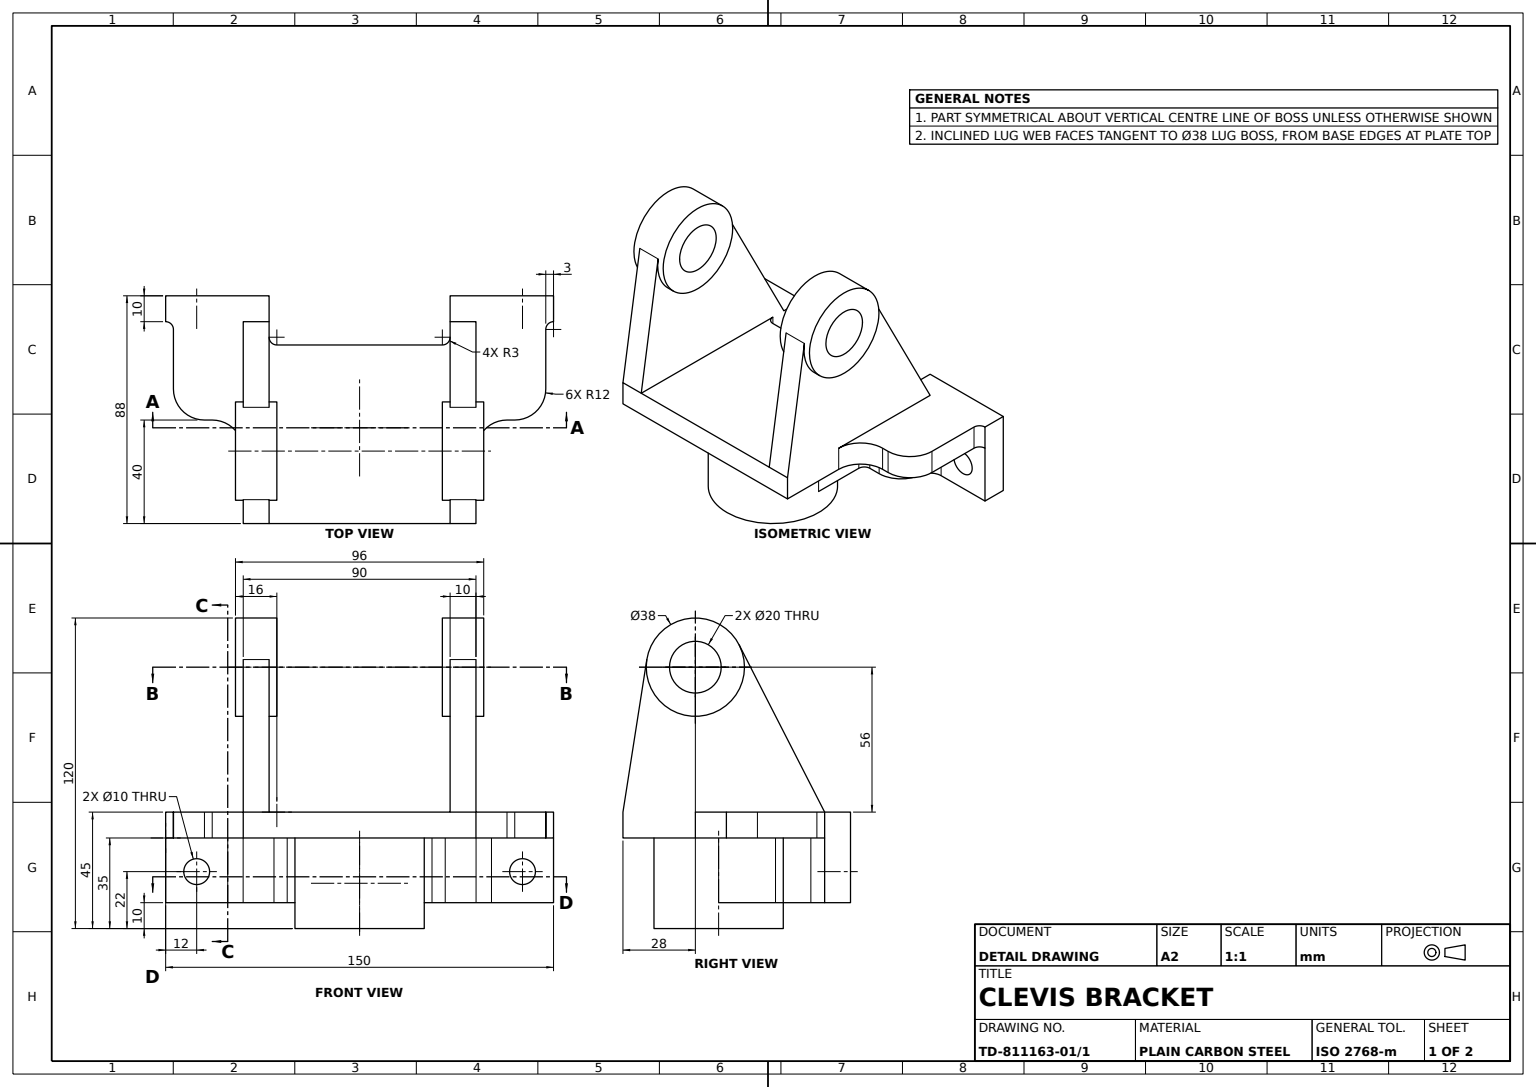
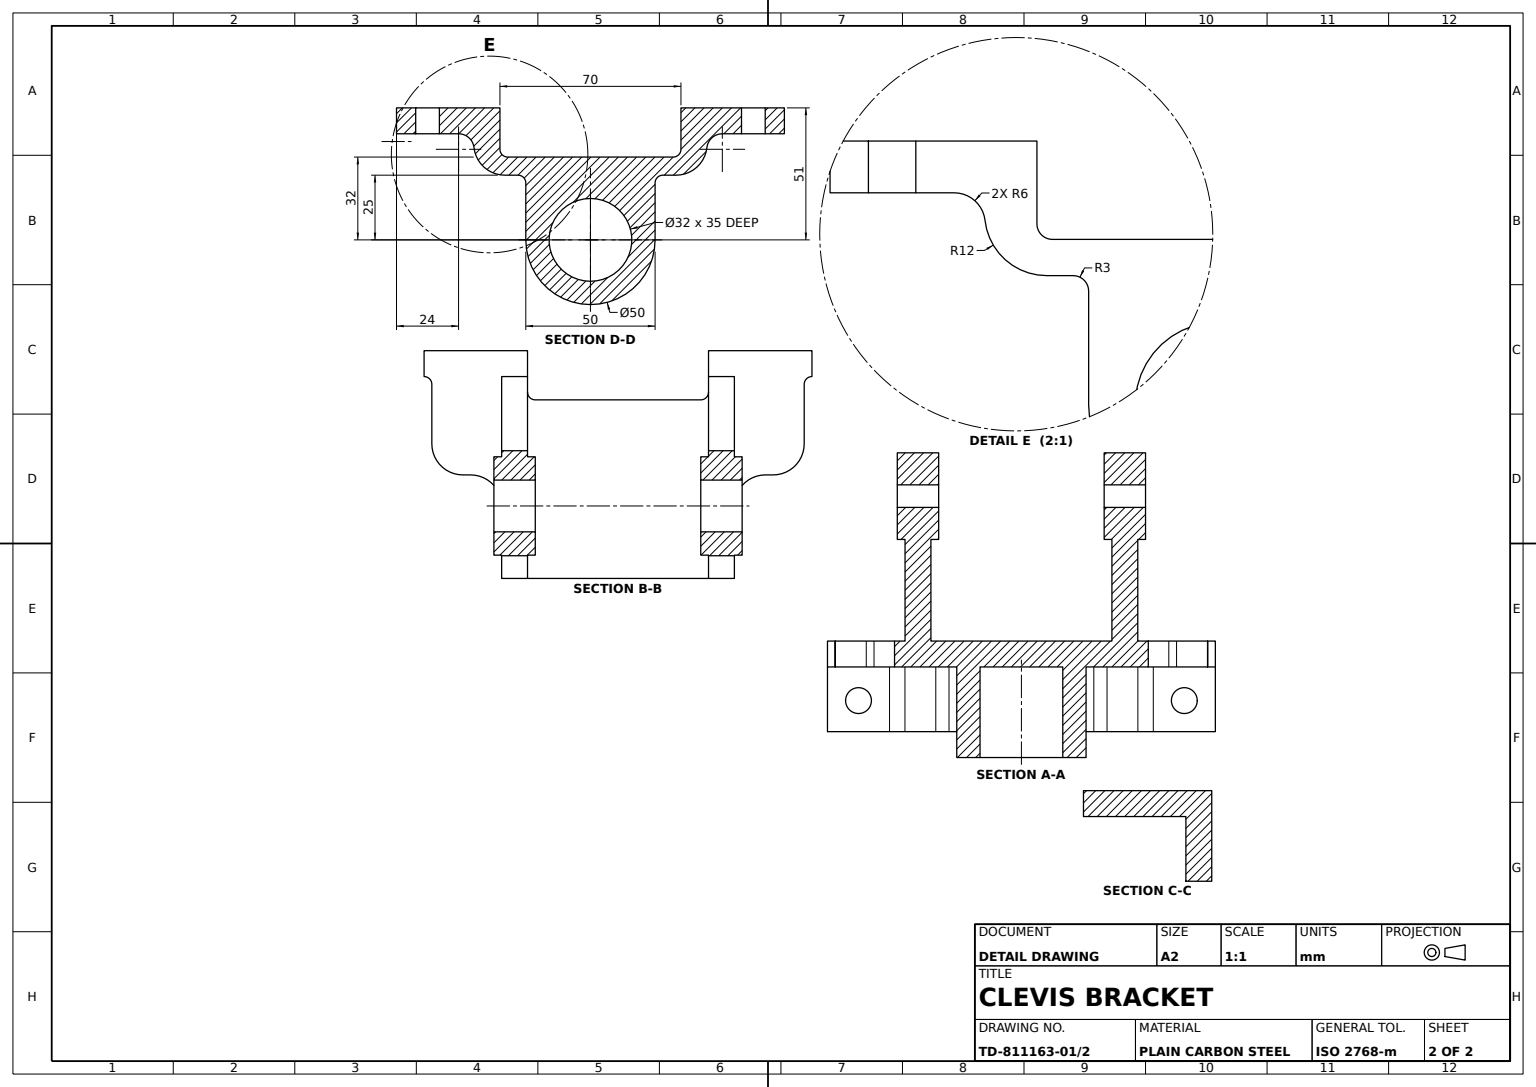
solid
v1 (48,101,19)
v2 (32,101,19)
e1 v1 v2 LINE
v3 (48,101,-1)
e2 v3 v1 CIRCLE(AX(P(48,101,9),D(-1,0,0),D(0,0,1)),10)
v4 (32,101,-1)
e3 v3 v4 LINE
e4 v4 v2 CIRCLE(AX(P(32,101,9),D(-1,0,0),D(0,0,1)),10)
face CYL(AX(P(75,101,9),D(-1,0,0),D(0,0,1)),10) rev [-e1 -e2 e3 e4]
v5 (-45.037152,10,-35.666667)
v6 (-45.037152,35,-35.666667)
e5 v5 v6 LINE
v7 (-51,35,-41)
e6 v7 v6 CIRCLE(AX(P(-51,35,-35),D(0,-1,0),D(0,0,1)),6)
v8 (-51,10,-41)
e7 v8 v7 LINE
e8 v8 v5 CIRCLE(AX(P(-51,10,-35),D(0,-1,0),D(0,0,1)),6)
face CYL(AX(P(-51,10,-35),D(0,1,0),D(0,0,1)),6) rev [e5 -e6 -e7 e8]
v9 (-68,22,-41)
v10 (-58,22,-41)
e9 v9 v10 CIRCLE(AX(P(-63,22,-41),D(0,0,1),D(1,0,0)),5)
e10 v10 v9 CIRCLE(AX(P(-63,22,-41),D(0,0,1),D(1,0,0)),5)
v11 (-75,10,-41)
e11 v11 v8 LINE
v12 (-75,35,-41)
e12 v12 v7 LINE
e13 v11 v12 LINE
face PLANE(AX(P(-51,10,-41),D(0,0,1),D(1,0,0))) [-e9 -e10] [e11 e7 -e12 -e13]
v13 (-48,101,-1)
v14 (-48,101,19)
e14 v13 v14 CIRCLE(AX(P(-48,101,9),D(-1,0,0),D(0,0,1)),10)
e15 v14 v13 CIRCLE(AX(P(-48,101,9),D(-1,0,0),D(0,0,1)),10)
v15 (-48,101,28)
v16 (-48,101,-10)
e16 v15 v16 CIRCLE(AX(P(-48,101,9),D(1,0,0),D(0,0,-1)),19)
e17 v16 v15 CIRCLE(AX(P(-48,101,9),D(1,0,0),D(0,0,-1)),19)
face PLANE(AX(P(-48,0,0),D(1,0,0),D(0,0,-1))) rev [-e14 -e15] [-e16 -e17]
v17 (32,45,-32)
v18 (-32,45,-32)
e18 v17 v18 LINE
v19 (-35,45,-35)
e19 v18 v19 CIRCLE(AX(P(-32,45,-35),D(0,-1,0),D(0,0,1)),3)
v20 (-35,45,37)
e20 v20 v19 LINE
v21 (35,45,37)
e21 v20 v21 LINE
v22 (35,45,-35)
e22 v21 v22 LINE
e23 v22 v17 CIRCLE(AX(P(32,45,-35),D(0,-1,0),D(0,0,1)),3)
face PLANE(AX(P(-57,45,9),D(0,-1,0),D(0,0,-1))) rev [e18 e19 -e20 e21 e22 e23]
v23 (-75,45,-41)
v24 (-72,45,-38)
e24 v23 v24 CIRCLE(AX(P(-75,45,-38),D(0,-1,0),D(0,0,-1)),3)
e25 v12 v23 LINE
v25 (-72,35,-38)
e26 v25 v12 CIRCLE(AX(P(-75,35,-38),D(0,1,0),D(0,0,-1)),3)
e27 v24 v25 LINE
face CYL(AX(P(-75,45,-38),D(0,-1,0),D(0,0,-1)),3) rev [-e24 -e25 -e26 -e27]
v26 (-25,10,0)
v27 (0,10,-25)
e28 v26 v27 CIRCLE(AX(P(0,10,0),D(0,-1,0),D(0,0,1)),25)
v28 (0,0,-25)
e29 v27 v28 LINE
v29 (0,0,25)
e30 v28 v29 CIRCLE(AX(P(0,0,0),D(0,1,0),D(0,0,1)),25)
v30 (0,35,25)
e31 v30 v29 LINE
v31 (-25,35,0)
e32 v31 v30 CIRCLE(AX(P(0,35,0),D(0,1,0),D(0,0,1)),25)
e33 v26 v31 LINE
face CYL(AX(P(0,35,0),D(0,-1,0),D(0,0,-1)),25) [e28 e29 e30 -e31 -e32 -e33]
v32 (28,10,-25)
v33 (33.111456,10,-25)
e34 v32 v33 LINE
v34 (33.111456,35,-25)
e35 v33 v34 LINE
v35 (28,35,-25)
e36 v35 v34 LINE
e37 v32 v35 LINE
face PLANE(AX(P(45,10,-25),D(0,0,1),D(1,0,0))) [e34 e35 -e36 -e37]
v36 (58,22,-51)
v37 (68,22,-51)
e38 v36 v37 CIRCLE(AX(P(63,22,-51),D(0,0,1),D(1,0,0)),5)
e39 v37 v36 CIRCLE(AX(P(63,22,-51),D(0,0,1),D(1,0,0)),5)
v38 (75,45,-51)
v39 (35,45,-51)
e40 v38 v39 LINE
v40 (75,10,-51)
e41 v40 v38 LINE
v41 (35,10,-51)
e42 v40 v41 LINE
e43 v41 v39 LINE
face PLANE(AX(P(35,10,-51),D(0,0,-1),D(-1,0,0))) [e38 e39] [-e40 -e41 e42 e43]
e44 v29 v28 CIRCLE(AX(P(0,0,0),D(0,1,0),D(0,0,1)),25)
v42 (0,0,-16)
v43 (0,0,16)
e45 v42 v43 CIRCLE(AX(P(0,0,0),D(0,-1,0),D(0,0,-1)),16)
e46 v43 v42 CIRCLE(AX(P(0,0,0),D(0,-1,0),D(0,0,-1)),16)
face PLANE(AX(P(0,0,0),D(0,1,0),D(0,0,1))) rev [-e30 -e44] [-e45 -e46]
v44 (-25,10,-22)
v45 (-25,35,-22)
e47 v44 v45 LINE
v46 (-28,35,-25)
e48 v46 v45 CIRCLE(AX(P(-28,35,-22),D(0,-1,0),D(0,0,1)),3)
v47 (-28,10,-25)
e49 v47 v46 LINE
e50 v47 v44 CIRCLE(AX(P(-28,10,-22),D(0,-1,0),D(0,0,1)),3)
face CYL(AX(P(-28,10,-22),D(0,1,0),D(0,0,1)),3) rev [e47 -e48 -e49 e50]
v48 (48,101,28)
v49 (48,101,-10)
e51 v48 v49 CIRCLE(AX(P(48,101,9),D(1,0,0),D(0,0,-1)),19)
e52 v49 v48 CIRCLE(AX(P(48,101,9),D(1,0,0),D(0,0,-1)),19)
e53 v1 v3 CIRCLE(AX(P(48,101,9),D(-1,0,0),D(0,0,1)),10)
face PLANE(AX(P(48,0,0),D(-1,0,0),D(0,0,-1))) rev [e51 e52] [e53 e2]
v50 (-35,10,-51)
v51 (-35,45,-51)
e54 v50 v51 LINE
v52 (-75,10,-51)
e55 v50 v52 LINE
v53 (-75,45,-51)
e56 v52 v53 LINE
e57 v51 v53 LINE
v54 (-68,22,-51)
v55 (-58,22,-51)
e58 v54 v55 CIRCLE(AX(P(-63,22,-51),D(0,0,1),D(1,0,0)),5)
e59 v55 v54 CIRCLE(AX(P(-63,22,-51),D(0,0,1),D(1,0,0)),5)
face PLANE(AX(P(-75,10,-51),D(0,0,-1),D(-1,0,0))) [-e54 e55 e56 -e57] [e58 e59]
v56 (-33.111456,10,-25)
e60 v56 v47 LINE
v57 (-33.111456,35,-25)
e61 v57 v46 LINE
e62 v57 v56 LINE
face PLANE(AX(P(-28,10,-25),D(0,0,1),D(1,0,0))) [e60 e49 -e61 e62]
v58 (68,22,-41)
v59 (58,22,-41)
e63 v58 v59 CIRCLE(AX(P(63,22,-41),D(0,0,1),D(1,0,0)),5)
e64 v59 v58 CIRCLE(AX(P(63,22,-41),D(0,0,1),D(1,0,0)),5)
v60 (51,10,-41)
v61 (51,35,-41)
e65 v60 v61 LINE
v62 (75,10,-41)
e66 v60 v62 LINE
v63 (75,35,-41)
e67 v62 v63 LINE
e68 v61 v63 LINE
face PLANE(AX(P(75,10,-41),D(0,0,1),D(1,0,0))) [-e63 -e64] [-e65 e66 e67 -e68]
v64 (72,35,-38)
v65 (72,45,-38)
e69 v64 v65 LINE
v66 (72,45,-15)
e70 v66 v65 LINE
v67 (72,35,-15)
e71 v66 v67 LINE
e72 v67 v64 LINE
face PLANE(AX(P(72,45,-41),D(-1,0,0),D(0,0,1))) rev [e69 -e70 e71 e72]
e73 v52 v11 LINE
e74 v53 v23 LINE
face PLANE(AX(P(-75,10,-41),D(-1,0,0),D(0,0,1))) [e73 e13 e25 -e74 -e56]
v68 (35,10,-35)
e75 v41 v68 LINE
e76 v68 v22 LINE
v69 (35,103.939212,27.771282)
e77 v21 v69 LINE
v70 (35,101,28)
e78 v69 v70 CIRCLE(AX(P(35,101,9),D(1,0,0),D(0,0,-1)),19)
v71 (35,101,-10)
e79 v70 v71 CIRCLE(AX(P(35,101,9),D(1,0,0),D(0,0,-1)),19)
v72 (35,109.655382,-7.914028)
e80 v71 v72 CIRCLE(AX(P(35,101,9),D(1,0,0),D(0,0,-1)),19)
v73 (35,45,-41)
e81 v73 v72 LINE
e82 v39 v73 LINE
face PLANE(AX(P(35,10,-35),D(-1,0,0),D(0,0,1))) [-e43 e75 e76 -e22 e77 e78 e79 e80 -e81 -e82]
e83 v45 v31 LINE
e84 v44 v26 LINE
face PLANE(AX(P(-25,10,0),D(-1,0,0),D(0,0,1))) [-e83 -e47 e84 e33]
v74 (-45,101,-10)
e85 v74 v16 LINE
v75 (-45,101,28)
e86 v75 v74 CIRCLE(AX(P(-45,101,9),D(1,0,0),D(0,0,-1)),19)
e87 v75 v15 LINE
face CYL(AX(P(-32,101,9),D(-1,0,0),D(0,0,1)),19) [-e85 -e86 e87 e16]
v76 (-57,45,-3)
v77 (-57,35,-3)
e88 v76 v77 LINE
v78 (-45,35,9)
e89 v77 v78 CIRCLE(AX(P(-57,35,9),D(0,-1,0),D(0,0,-1)),12)
v79 (-45,45,9)
e90 v79 v78 LINE
e91 v76 v79 CIRCLE(AX(P(-57,45,9),D(0,-1,0),D(0,0,-1)),12)
face CYL(AX(P(-57,45,9),D(0,-1,0),D(0,0,-1)),12) rev [e88 e89 -e90 -e91]
e92 v36 v59 LINE
e93 v37 v58 LINE
face CYL(AX(P(63,22,-51),D(0,0,1),D(1,0,0)),5) rev [-e92 -e39 e93 e63]
v80 (-45,45,37)
v81 (-45,103.939212,27.771282)
e94 v80 v81 LINE
e95 v80 v20 LINE
v82 (-35,103.939212,27.771282)
e96 v20 v82 LINE
e97 v82 v81 LINE
face PLANE(AX(P(-35,6.731708,42.99206),D(0,0.154695393,0.987962214),D(0,-0.987962214,0.154695393))) [-e94 e95 e96 e97]
v83 (-35,10,-35)
e98 v83 v19 LINE
e99 v83 v50 LINE
v84 (-35,45,-41)
e100 v84 v51 LINE
v85 (-35,109.655382,-7.914028)
e101 v84 v85 LINE
v86 (-35,101,-10)
e102 v86 v85 CIRCLE(AX(P(-35,101,9),D(1,0,0),D(0,0,-1)),19)
v87 (-35,101,28)
e103 v87 v86 CIRCLE(AX(P(-35,101,9),D(1,0,0),D(0,0,-1)),19)
e104 v82 v87 CIRCLE(AX(P(-35,101,9),D(1,0,0),D(0,0,-1)),19)
face PLANE(AX(P(-35,10,-51),D(1,0,0),D(0,0,-1))) [-e96 e20 -e98 e99 e54 -e100 e101 -e102 -e103 -e104]
v88 (25,10,-22)
v89 (25,35,-22)
e105 v88 v89 LINE
v90 (25,35,0)
e106 v90 v89 LINE
v91 (25,10,0)
e107 v91 v90 LINE
e108 v91 v88 LINE
face PLANE(AX(P(25,10,-22),D(1,0,0),D(0,0,-1))) [e105 -e106 -e107 e108]
v92 (0,35,-16)
e109 v92 v42 LINE
v93 (0,35,16)
e110 v93 v43 LINE
e111 v93 v92 CIRCLE(AX(P(0,35,0),D(0,1,0),D(0,0,-1)),16)
face CYL(AX(P(0,45,0),D(0,-1,0),D(0,0,-1)),16) rev [e109 e45 -e110 e111]
e112 v92 v93 CIRCLE(AX(P(0,35,0),D(0,1,0),D(0,0,-1)),16)
face CYL(AX(P(0,45,0),D(0,-1,0),D(0,0,-1)),16) rev [e112 e110 e46 -e109]
e113 v6 v57 CIRCLE(AX(P(-33.111456,35,-37),D(0,1,0),D(0,0,-1)),12)
e114 v56 v5 CIRCLE(AX(P(-33.111456,10,-37),D(0,-1,0),D(0,0,1)),12)
face CYL(AX(P(-33.111456,10,-37),D(0,1,0),D(0,0,1)),12) [-e62 -e113 -e5 -e114]
v94 (45,45,-41)
e115 v73 v94 LINE
v95 (45,109.655382,-7.914028)
e116 v72 v95 LINE
e117 v94 v95 LINE
face PLANE(AX(P(35,25.965365,-50.740556),D(0,0.455546445,-0.890212018),D(0,0.890212018,0.455546445))) [-e115 e81 e116 -e117]
v96 (45.037152,10,-35.666667)
e118 v96 v60 CIRCLE(AX(P(51,10,-35),D(0,-1,0),D(0,0,1)),6)
e119 v96 v33 CIRCLE(AX(P(33.111456,10,-37),D(0,-1,0),D(0,0,1)),12)
e120 v88 v32 CIRCLE(AX(P(28,10,-22),D(0,-1,0),D(0,0,-1)),3)
e121 v27 v91 CIRCLE(AX(P(0,10,0),D(0,-1,0),D(0,0,1)),25)
v97 (-32,10,-32)
e122 v97 v83 CIRCLE(AX(P(-32,10,-35),D(0,-1,0),D(0,0,1)),3)
v98 (32,10,-32)
e123 v98 v97 LINE
e124 v68 v98 CIRCLE(AX(P(32,10,-35),D(0,-1,0),D(0,0,1)),3)
e125 v62 v40 LINE
face PLANE(AX(P(0,10,0),D(0,1,0),D(0,0,1))) rev [-e66 -e118 e119 -e34 -e120 -e108 -e121 -e28 -e84 -e50 -e60 e114 -e8 -e11 -e73 -e55 -e99 -e122 -e123 -e124 -e75 -e42 -e125]
v99 (32,101,28)
e126 v99 v70 LINE
v100 (32,101,-10)
e127 v99 v100 CIRCLE(AX(P(32,101,9),D(1,0,0),D(0,0,-1)),19)
e128 v100 v71 LINE
face CYL(AX(P(32,101,9),D(1,0,0),D(0,0,-1)),19) [-e79 -e126 e127 e128]
v101 (-32,101,-1)
e129 v101 v13 LINE
v102 (-32,101,19)
e130 v101 v102 CIRCLE(AX(P(-32,101,9),D(1,0,0),D(0,0,-1)),10)
e131 v102 v14 LINE
face CYL(AX(P(75,101,9),D(-1,0,0),D(0,0,1)),10) rev [e15 -e129 e130 e131]
v103 (45,103.939212,27.771282)
e132 v69 v103 LINE
v104 (45,101,28)
e133 v103 v104 CIRCLE(AX(P(45,101,9),D(1,0,0),D(0,0,-1)),19)
e134 v104 v48 LINE
v105 (45,101,-10)
e135 v105 v49 LINE
e136 v105 v95 CIRCLE(AX(P(45,101,9),D(1,0,0),D(0,0,-1)),19)
e137 v100 v99 CIRCLE(AX(P(32,101,9),D(1,0,0),D(0,0,-1)),19)
face CYL(AX(P(32,101,9),D(1,0,0),D(0,0,-1)),19) [e132 e133 e134 -e52 -e135 e136 -e116 -e80 -e128 e137 e126 -e78]
e138 v54 v9 LINE
e139 v55 v10 LINE
face CYL(AX(P(-63,22,-51),D(0,0,1),D(1,0,0)),5) rev [-e138 -e59 e139 e10]
v106 (57,45,-3)
v107 (57,35,-3)
e140 v106 v107 LINE
v108 (60,35,-3)
e141 v107 v108 LINE
v109 (60,45,-3)
e142 v109 v108 LINE
e143 v106 v109 LINE
face PLANE(AX(P(60,45,-3),D(0,0,-1),D(-1,0,0))) rev [e140 e141 -e142 -e143]
v110 (-32,101,-10)
e144 v110 v86 LINE
v111 (-32,101,28)
e145 v111 v110 CIRCLE(AX(P(-32,101,9),D(1,0,0),D(0,0,-1)),19)
e146 v111 v87 LINE
face CYL(AX(P(-32,101,9),D(-1,0,0),D(0,0,1)),19) [e103 -e144 -e145 e146]
v112 (45.037152,35,-35.666667)
e147 v112 v61 CIRCLE(AX(P(51,35,-35),D(0,-1,0),D(0,0,1)),6)
e148 v112 v96 LINE
face CYL(AX(P(51,10,-35),D(0,1,0),D(0,0,1)),6) rev [e118 e65 -e147 e148]
face CYL(AX(P(63,22,-51),D(0,0,1),D(1,0,0)),5) rev [e92 e64 -e93 -e38]
e149 v104 v105 CIRCLE(AX(P(45,101,9),D(1,0,0),D(0,0,-1)),19)
v113 (45,45,37)
e150 v113 v103 LINE
v114 (45,35,37)
e151 v113 v114 LINE
v115 (45,35,9)
e152 v114 v115 LINE
v116 (45,45,9)
e153 v116 v115 LINE
e154 v116 v94 LINE
face PLANE(AX(P(45,45,9),D(-1,0,0),D(0,0,1))) rev [e117 -e136 -e149 -e133 -e150 e151 e152 -e153 e154]
e155 v34 v112 CIRCLE(AX(P(33.111456,35,-37),D(0,1,0),D(0,0,-1)),12)
face CYL(AX(P(33.111456,10,-37),D(0,1,0),D(0,0,1)),12) [-e148 -e155 -e35 -e119]
e156 v98 v17 LINE
face CYL(AX(P(32,10,-35),D(0,1,0),D(0,0,1)),3) rev [-e76 e124 e156 -e23]
v117 (-72,45,-15)
v118 (-60,45,-3)
e157 v117 v118 CIRCLE(AX(P(-60,45,-15),D(0,1,0),D(0,0,1)),12)
e158 v118 v76 LINE
v119 (-45,45,-41)
e159 v79 v119 LINE
e160 v84 v119 LINE
e161 v24 v117 LINE
face PLANE(AX(P(-57,45,9),D(0,-1,0),D(0,0,-1))) rev [e157 e158 e91 e159 -e160 e100 e57 e74 e24 e161]
v120 (75,45,-41)
e162 v63 v120 LINE
e163 v65 v120 CIRCLE(AX(P(75,45,-38),D(0,-1,0),D(0,0,-1)),3)
e164 v63 v64 CIRCLE(AX(P(75,35,-38),D(0,1,0),D(0,0,-1)),3)
face CYL(AX(P(75,10,-38),D(0,-1,0),D(0,0,-1)),3) rev [e162 -e163 -e69 -e164]
e165 v110 v111 CIRCLE(AX(P(-32,101,9),D(1,0,0),D(0,0,-1)),19)
e166 v102 v101 CIRCLE(AX(P(-32,101,9),D(1,0,0),D(0,0,-1)),10)
face PLANE(AX(P(-32,0,0),D(1,0,0),D(0,0,-1))) [e165 e145] [-e166 -e130]
v121 (-45,109.655382,-7.914028)
e167 v74 v121 CIRCLE(AX(P(-45,101,9),D(1,0,0),D(0,0,-1)),19)
e168 v119 v121 LINE
v122 (-45,35,37)
e169 v78 v122 LINE
e170 v80 v122 LINE
e171 v81 v75 CIRCLE(AX(P(-45,101,9),D(1,0,0),D(0,0,-1)),19)
face PLANE(AX(P(-45,45,9),D(1,0,0),D(0,0,-1))) rev [e167 -e168 -e159 e90 e169 -e170 e94 e171 e86]
face CYL(AX(P(32,101,9),D(1,0,0),D(0,0,-1)),19) [e149 e135 -e51 -e134]
e172 v116 v106 CIRCLE(AX(P(57,45,9),D(0,-1,0),D(0,0,1)),12)
e173 v115 v107 CIRCLE(AX(P(57,35,9),D(0,-1,0),D(0,0,1)),12)
face CYL(AX(P(57,45,9),D(0,-1,0),D(0,0,-1)),12) rev [-e140 -e172 e153 e173]
e174 v120 v38 LINE
face PLANE(AX(P(75,10,-51),D(1,0,0),D(0,0,-1))) [-e174 -e162 -e67 e125 e41]
face CYL(AX(P(75,101,9),D(-1,0,0),D(0,0,1)),10) rev [e129 e14 -e131 e166]
face CYL(AX(P(-63,22,-51),D(0,0,1),D(1,0,0)),5) rev [e9 -e139 -e58 e138]
e175 v89 v35 CIRCLE(AX(P(28,35,-22),D(0,-1,0),D(0,0,-1)),3)
face CYL(AX(P(28,10,-22),D(0,1,0),D(0,0,1)),3) rev [-e105 e120 e37 -e175]
e176 v21 v113 LINE
face PLANE(AX(P(35,6.731708,42.99206),D(0,-0.154695393,-0.987962214),D(0,0.987962214,-0.154695393))) rev [-e77 e176 e150 -e132]
e177 v97 v18 LINE
face CYL(AX(P(-32,10,-35),D(0,1,0),D(0,0,1)),3) rev [e122 e98 -e19 -e177]
e178 v109 v66 CIRCLE(AX(P(60,45,-15),D(0,1,0),D(0,0,-1)),12)
e179 v108 v67 CIRCLE(AX(P(60,35,-15),D(0,1,0),D(0,0,-1)),12)
face CYL(AX(P(60,45,-15),D(0,-1,0),D(0,0,-1)),12) [-e71 -e178 e142 e179]
e180 v85 v121 LINE
face CYL(AX(P(-32,101,9),D(-1,0,0),D(0,0,1)),19) [-e171 -e97 e104 -e146 -e165 e144 e102 e180 -e167 e85 e17 -e87]
v123 (-60,35,-3)
e181 v123 v77 LINE
v124 (-72,35,-15)
e182 v124 v123 CIRCLE(AX(P(-60,35,-15),D(0,1,0),D(0,0,1)),12)
e183 v25 v124 LINE
e184 v30 v90 CIRCLE(AX(P(0,35,0),D(0,1,0),D(0,0,1)),25)
e185 v122 v114 LINE
face PLANE(AX(P(-57,35,9),D(0,-1,0),D(0,0,-1))) [-e181 -e182 -e183 e26 e12 e6 e113 e61 e48 e83 e32 e184 e106 e175 e36 e155 e147 e68 e164 -e72 -e179 -e141 -e173 -e152 -e185 -e169 -e89]
e186 v117 v124 LINE
face PLANE(AX(P(-72,45,-41),D(1,0,0),D(0,0,-1))) rev [-e161 e27 e183 -e186]
e187 v2 v4 CIRCLE(AX(P(32,101,9),D(-1,0,0),D(0,0,1)),10)
face CYL(AX(P(75,101,9),D(-1,0,0),D(0,0,1)),10) rev [e187 -e3 -e53 e1]
face PLANE(AX(P(-57,45,9),D(0,-1,0),D(0,0,-1))) rev [e115 -e154 e172 e143 e178 e70 e163 e174 e40 e82]
face PLANE(AX(P(-45,45,37),D(0,0,-1),D(-1,0,0))) rev [-e176 -e21 -e95 e170 e185 -e151]
face PLANE(AX(P(57,35,9),D(0,-1,0),D(0,0,-1))) [-e111 -e112]
face PLANE(AX(P(-35,25.965365,-50.740556),D(0,-0.455546445,0.890212018),D(0,-0.890212018,-0.455546445))) rev [-e180 -e101 e160 e168]
face PLANE(AX(P(-32,10,-32),D(0,0,-1),D(-1,0,0))) [-e18 -e156 e123 e177]
e188 v118 v123 LINE
face PLANE(AX(P(-60,45,-3),D(0,0,-1),D(-1,0,0))) rev [e181 -e88 -e158 e188]
face CYL(AX(P(-60,45,-15),D(0,-1,0),D(0,0,-1)),12) [-e188 -e157 e186 e182]
face PLANE(AX(P(32,0,0),D(-1,0,0),D(0,0,-1))) [-e137 -e127] [-e4 -e187]
face CYL(AX(P(0,35,0),D(0,-1,0),D(0,0,-1)),25) [-e29 e121 e107 -e184 e31 e44]
